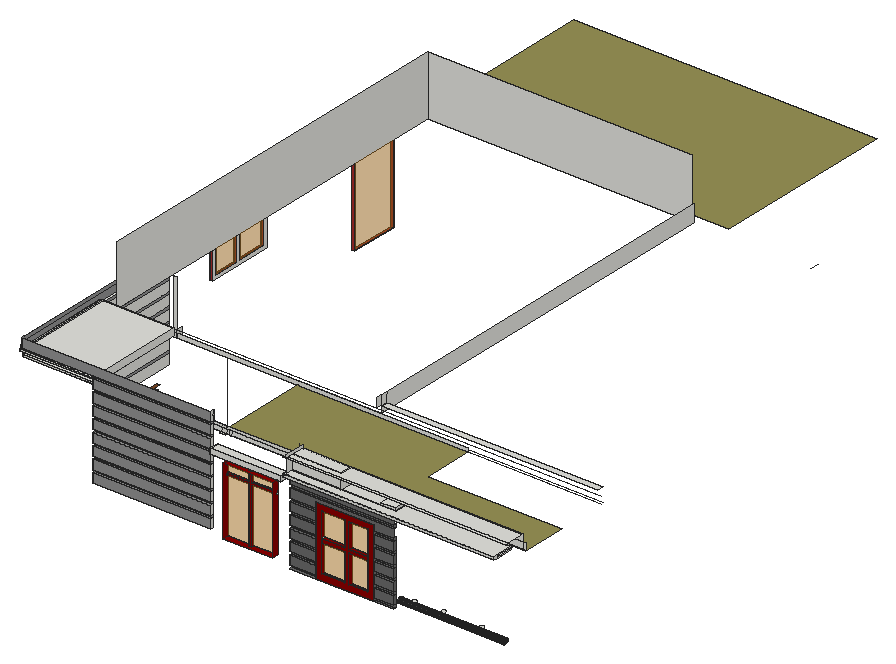
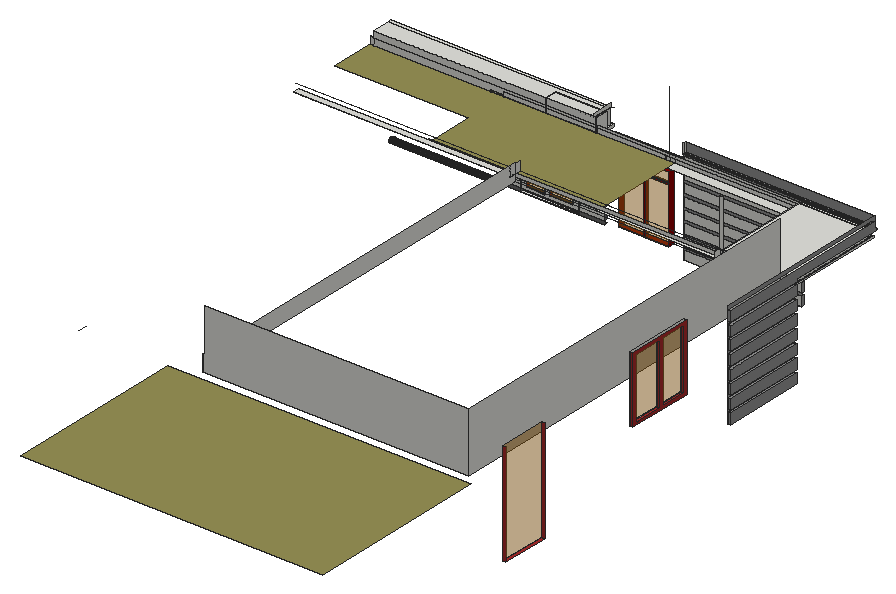
# SketchUp Ruby script. Lengths in inches.
U = 1.inch
M = Sketchup.active_model
def pt(a) = Geom::Point3d.new(a.map { |v| v * U })
def face(e, loops, mat)
  f = e.add_face(loops[0].map { |a| pt(a) })
  loops[1..].each { |l| e.add_face(l.map { |a| pt(a) }).erase! }
  f.material = f.back_material = mat if mat
  f
end
# faces: each face lists its corners as indices into pts; further lists are holes
def faces(e, pts, list, mat = nil) = list.each { |f| face(e, (f[0].is_a?(Array) ? f : [f]).map { |l| l.map { |i| pts[i] } }, mat) }
# xy, xz, yz: faces in a plane at the given z, y or x. An outline is a flat list of corners, or four numbers for a rectangle; further outlines are holes
def ring(l) = l.size == 4 ? [[l[0], l[1]], [l[2], l[1]], [l[2], l[3]], [l[0], l[3]]] : l.each_slice(2).to_a
def flat(e, list, mat, &to3) = list.each { |f| face(e, (f[0].is_a?(Array) ? f : [f]).map { |l| ring(l).map { |u, v| to3.(u, v) } }, mat) }
def xy(e, z, list, mat = nil) = flat(e, list, mat) { |x, y| [x, y, z] }
def xz(e, y, list, mat = nil) = flat(e, list, mat) { |x, z| [x, y, z] }
def yz(e, x, list, mat = nil) = flat(e, list, mat) { |y, z| [x, y, z] }
def lines(e, pts, list) = list.each { |a, b| e.add_line(pt(pts[a]), pt(pts[b])) }
# prism: a flat outline (further loops are holes) pulled along v
def prism(e, loops, v, mat = nil)
  f = face(e, loops, mat); d = Geom::Vector3d.new(v.map { |x| x * U })
  f.pushpull(f.normal.samedirection?(d) ? d.length : -d.length)
end
def box(e, o, s, mat = nil) = prism(e, [[o, [o[0] + s[0], o[1], o[2]], [o[0] + s[0], o[1] + s[1], o[2]], [o[0], o[1] + s[1], o[2]]]], [0, 0, s[2]], mat)
def at(x, y, z, deg = 0) = Geom::Transformation.translation(pt([x, y, z])) * Geom::Transformation.rotation(ORIGIN, Z_AXIS, deg.degrees)
def axes(o, x, y, z) = Geom::Transformation.new([*x, 0, *y, 0, *z, 0, *pt(o).to_a, 1])
def part(name) = M.definitions.add(name)
# library, detail: a bought-in or finely detailed component or shape, given as its bounding box
def library(name, o, s) = part(name).tap { |d| box(d.entities, o, s) }
def detail(e, o, s) = box(e.add_group.entities, o, s)
def put(e, d, t, mat = nil) = e.add_instance(d, t).tap { |i| i.material = mat if mat }
def group(e, t, mat = nil) = e.add_group.tap { |g| g.transformation = t; g.material = mat if mat }.entities
root = M.entities
M.materials.add("[0018_Brown]").color = [165, 42, 42]
M.materials.add("[0021_DarkRed]").color = [139, 0, 0]
M.materials.add("[0038_Orange]").color = [255, 165, 0]
M.materials.add("[0057_DarkKhaki]").color = [150, 145, 85]
M.materials.add("[0134_DimGray]").color = [105, 105, 105]
M.materials.add("[0137_Black]").color = [71, 71, 71]
M.materials.add("[Color M05]").color = [145, 145, 145]
M.materials.add("[Translucent Glass Gray]").color = [191, 123, 24]
M.materials["[Translucent Glass Gray]"].alpha = 0.5
M.materials.add("[Wood Veneer 01]").color = [120, 70, 37]
xy(root,274.6875,[[286.17,7.0625,335.53,10.0625],[335.53,7.0625,390.0625,10.0625]],"[0134_DimGray]")
xy(root,274.97,[[312.43,7.0625,370.43,10.0625]])
xy(root,276.08,[[8.875,431.78,11.875,479.72]],"[0018_Brown]")
xy(root,276.32,[[8.875,116.75,11.875,199.5]],"[Color M05]")
xy(root,276.55,[[82.85,15.1875,200.79,18.1875]])
xy(root,278.27,[[370.43,7.0625,390.0625,10.0625]])
xy(root,278.27,[[286.17,7.0625,312.43,10.0625]],"[0134_DimGray]")
xy(root,278.86,[[242.99,10.1875,245.59,12.1875]])
xy(root,278.86,[[220.5625,6.1875,270.625,6.1875,270.625,12.1875,245.59,12.1875,245.59,10.1875,242.99,10.1875,242.99,12.1875,220.5625,12.1875]],"[0021_DarkRed]")
xy(root,280.97,[[318.43,7.0625,341.43,10.0625],[345.85,7.0625,364.43,10.0625]],"[0021_DarkRed]")
xy(root,285.65,[[82.85,15.1875,200.79,18.1875]],"[Color M05]")
xy(root,286.4,[[8.875,116.75,11.875,199.5]],"[Color M05]")
xy(root,286.45,[[407.42,9.5,407.89,9.5625,408.33,9.74,408.7,10.03,408.99,10.41,409.17,10.84,409.23,11.3125,409.17,11.78,408.99,12.22,408.7,12.6,408.33,12.88,407.89,13.0625,407.42,13.125,406.95,13.0625,406.51,12.88,406.14,12.6,405.85,12.22,405.67,11.78,405.61,11.3125,405.67,10.84,405.85,10.41,406.14,10.03,406.51,9.74,406.95,9.5625]])
xy(root,286.6875,[[286.17,7.0625,312.43,10.0625],[370.43,7.0625,390.0625,10.0625]],"[0134_DimGray]")
xy(root,287.08,[[474.86,9.5,475.33,9.5625,475.76,9.74,476.14,10.03,476.43,10.41,476.61,10.84,476.67,11.3125,476.61,11.78,476.43,12.22,476.14,12.6,475.76,12.88,475.33,13.0625,474.86,13.125,474.39,13.0625,473.95,12.88,473.58,12.6,473.29,12.22,473.11,11.78,473.04,11.3125,473.11,10.84,473.29,10.41,473.58,10.03,473.95,9.74,474.39,9.5625]])
xy(root,287.52,[[437.11,9.5,437.58,9.5625,438.01,9.74,438.39,10.03,438.68,10.41,438.86,10.84,438.92,11.3125,438.86,11.78,438.68,12.22,438.39,12.6,438.01,12.88,437.58,13.0625,437.11,13.125,436.64,13.0625,436.2,12.88,435.83,12.6,435.54,12.22,435.36,11.78,435.29,11.3125,435.36,10.84,435.54,10.41,435.83,10.03,436.2,9.74,436.64,9.5625]])
xy(root,288.55,[[82.85,15.1875,200.79,18.1875]])
xy(root,289.44,[[8.875,116.75,11.875,199.5]],"[Color M05]")
xy(root,290.27,[[370.43,7.0625,390.0625,10.0625]])
xy(root,290.27,[[286.17,7.0625,312.43,10.0625]],"[0134_DimGray]")
xy(root,297.65,[[82.85,15.1875,200.79,18.1875]],"[Color M05]")
xy(root,298.6875,[[286.17,7.0625,312.43,10.0625],[370.43,7.0625,390.0625,10.0625]],"[0134_DimGray]")
xy(root,299.53,[[8.875,116.75,11.875,199.5]],"[Color M05]")
xy(root,300.55,[[82.85,15.1875,200.79,18.1875]])
xy(root,302.27,[[286.17,7.0625,312.43,10.0625],[370.43,7.0625,390.0625,10.0625]],"[0134_DimGray]")
xy(root,302.57,[[8.875,116.75,11.875,199.5]],"[Color M05]")
xy(root,309.43,[[318.43,7.0625,341.43,10.0625],[345.85,7.0625,364.43,10.0625]])
xy(root,309.65,[[82.85,15.1875,200.79,18.1875]],"[Color M05]")
xy(root,310.6875,[[286.17,7.0625,312.43,10.0625],[370.43,7.0625,390.0625,10.0625]],"[0134_DimGray]")
xy(root,312.55,[[82.85,15.1875,200.79,18.1875]])
xy(root,312.65,[[8.875,116.75,11.875,199.5]],"[Color M05]")
xy(root,312.85,[[318.43,7.0625,341.43,10.0625],[345.85,7.0625,364.43,10.0625]],"[0021_DarkRed]")
xy(root,314.27,[[286.17,7.0625,312.43,10.0625],[370.43,7.0625,390.0625,10.0625]],"[0134_DimGray]")
xy(root,315.69,[[8.875,116.75,11.875,199.5]],"[Color M05]")
xy(root,321.65,[[82.85,15.1875,200.79,18.1875]],"[Color M05]")
xy(root,322.6875,[[286.17,7.0625,312.43,10.0625],[370.43,7.0625,390.0625,10.0625]],"[0134_DimGray]")
xy(root,324,[[79.85,66.65,82.85,96.65]])
xy(root,324.55,[[82.85,15.1875,200.79,18.1875]],"[Color M05]")
xy(root,325.78,[[8.875,116.75,11.875,199.5]],"[Color M05]")
xy(root,326.27,[[286.17,7.0625,312.43,10.0625],[370.43,7.0625,390.0625,10.0625]],"[0134_DimGray]")
xy(root,327,[[79.85,63.65,82.85,99.65]],"[Wood Veneer 01]")
xy(root,327.4,[[8.875,254.47,11.875,321.35]],"[0018_Brown]")
xy(root,328.82,[[8.875,116.75,11.875,199.5]],"[Color M05]")
xy(root,330.4,[[8.875,257.47,11.875,284.61],[8.875,287.91,11.875,318.35]],"[0018_Brown]")
xy(root,333.65,[[82.85,15.1875,200.79,18.1875]],"[Color M05]")
xy(root,334.3,[[220.5625,10.1875,242.99,12.1875],[245.59,10.1875,270.625,12.1875]],"[0021_DarkRed]")
xy(root,334.6875,[[286.17,7.0625,312.43,10.0625],[370.43,7.0625,390.0625,10.0625]],"[0134_DimGray]")
xy(root,336.28,[[220.5625,10.1875,242.99,12.1875],[245.59,10.1875,270.625,12.1875]],"[0021_DarkRed]")
xy(root,336.55,[[82.85,15.1875,200.79,18.1875]],"[Color M05]")
xy(root,337.9,[[318.43,7.0625,341.43,10.0625],[345.85,7.0625,364.43,10.0625]])
xy(root,338.27,[[286.17,7.0625,312.43,10.0625],[370.43,7.0625,390.0625,10.0625]],"[0134_DimGray]")
xy(root,338.9,[[8.875,116.75,11.875,199.5]],"[Color M05]")
xy(root,341.94,[[8.875,116.75,11.875,199.5]],"[Color M05]")
xy(root,343.9,[[312.43,7.0625,370.43,10.0625]])
xy(root,345.65,[[82.85,15.1875,200.79,18.1875]],"[Color M05]")
xy(root,346.36,[[242.99,10.1875,245.59,12.1875]])
xy(root,346.36,[[220.5625,6.1875,220.5625,12.1875,242.99,12.1875,242.99,10.1875,245.59,10.1875,245.59,12.1875,270.625,12.1875,270.625,6.1875]],"[0021_DarkRed]")
xy(root,346.6875,[[286.17,7.0625,390.0625,10.0625]],"[0134_DimGray]")
xy(root,348.55,[[82.85,15.1875,200.79,18.1875]],"[Color M05]")
xy(root,350.27,[[286.17,7.0625,390.0625,10.0625]],"[0134_DimGray]")
xy(root,352.03,[[8.875,116.75,11.875,199.5]],"[Color M05]")
xy(root,352.16,[[209.95,3.1875,214.5625,12.1875],[276.625,3.1875,278.01,12.1875],[278.01,3.1875,280.45,12.1875],[280.45,3.1875,280.75,12.1875]])
xy(root,352.36,[[214.5625,3.1875,276.625,6.1875],[214.5625,6.1875,276.625,12.1875]])
xy(root,355.07,[[8.875,116.75,11.875,199.5]])
xy(root,357.35,[[209.95,3.1875,280.45,12.1875]])
xy(root,357.65,[[82.85,15.1875,200.79,18.1875]],"[Color M05]")
xy(root,358.6875,[[284.41,1.0625,284.41,10.0625,286.17,10.0625,286.17,7.0625,390.0625,7.0625,390.0625,22.0625,495.71,22.0625,495.71,1.0625],[286.17,7.0625,286.99,10.0625],[286.99,7.0625,335.53,10.0625],[335.53,7.0625,375.29,10.0625],[375.29,7.0625,390.0625,10.0625],
  [284.41,10.0625,335.53,22.0625],[335.53,10.0625,390.0625,22.0625]])
xy(root,360.55,[[82.85,15.1875,200.79,18.1875]],"[Color M05]")
xy(root,361.64,[[285.64,4.0625,497.49,22.0625]])
xy(root,361.6875,[[284.41,1.0625,495.71,1.0625,495.71,22.0625,390.0625,22.0625,390.0625,10.0625,284.41,10.0625]])
xy(root,363,[[206.66,19.6875,211.87,22.0625],[211.87,21.8125,216.79,22.0625],[86.03,22.0625,206.66,31.8125],[86.03,116.75,206.66,119.6875]])
xy(root,363,[[206.66,22.0625,206.66,116.75,376.99,116.75,376.99,66.25,510.6875,66.25,510.6875,22.0625],[11.875,520.875,314.375,705.1875]],"[0057_DarkKhaki]")
xy(root,363.17,[[11.875,22.0625,20.6875,32.5]])
xy(root,363.37,[[10.5625,18.1875,82.85,116.75]])
xy(root,363.92,[[375.29,10.0625,390.0625,22.0625]])
xy(root,364.96,[[10.5625,18.1875,82.85,18.1875,82.85,21.1875,11.875,21.1875,11.875,116.75,10.5625,116.75]])
xy(root,365.15,[[8.875,116.75,11.875,199.5]],"[Color M05]")
xy(root,368.19,[[8.875,116.75,11.875,199.5]])
xy(root,369.18,[[10.1875,15.5625,10.1875,116.75,11.875,116.75,11.875,21.1875,82.85,21.1875,82.85,15.5625]])
xy(root,369.65,[[82.85,15.1875,200.79,18.1875]],"[Color M05]")
xy(root,369.99,[[285.29,122.75,286.17,128.75],[286.17,122.75,501.6875,128.75]])
xy(root,370.55,[[10.1875,15.5625,82.85,18.1875],[8.875,18.1875,10.1875,116.75],[10.1875,18.1875,11.875,21.1875],[11.875,18.1875,82.85,21.1875],[10.1875,21.1875,11.875,21.75],
  [11.875,21.1875,82.85,21.75],[10.1875,21.75,11.875,116.75],[11.875,21.75,82.85,116.75]])
xy(root,372.55,[[8.875,18.1875,11.875,19],[11.875,18.1875,200.79,19]])
xy(root,372.55,[[11.875,15.1875,200.79,18.1875]],"[Color M05]")
xy(root,376.42,[[286.99,1.0625,507.04,4.0625],[285.64,4.0625,286.99,10.0625],[286.99,4.0625,507.04,4.0625,507.04,22.0625,335.53,22.0625,335.53,10.0625,286.99,10.0625],[284.41,10.0625,285.64,22.0625],[285.64,10.0625,286.99,22.0625],
  [286.99,10.0625,335.53,22.0625]])
xz(root,1.0625,[[284.41,358.6875,495.71,361.64],[284.41,361.64,285.29,361.6875],[285.29,361.64,286.17,361.6875],[286.17,361.64,286.99,361.6875],[286.99,361.64,495.71,361.6875]])
xz(root,3.1875,[[209.95,352.16,214.5625,352.16,214.5625,352.36,276.625,352.36,276.625,352.16,280.45,352.16,280.45,357.35,209.95,357.35]])
xz(root,7.0625,[[[312.43,274.97,370.43,343.9],[318.43,280.97,318.43,337.9,341.43,337.9,341.43,312.85,318.43,312.85,318.43,309.43,341.43,309.43,341.43,280.97],[345.85,280.97,345.85,309.43,364.43,309.43,364.43,312.85,345.85,312.85,345.85,337.9,364.43,337.9,364.43,280.97]]],"[0021_DarkRed]")
xz(root,7.0625,[[286.17,278.27,312.43,286.6875],[370.43,278.27,390.0625,286.6875],[286.17,290.27,312.43,298.6875],[370.43,290.27,390.0625,298.6875],[286.17,302.27,312.43,310.6875],
  [370.43,302.27,390.0625,310.6875],[286.17,314.27,312.43,322.6875],[370.43,314.27,390.0625,322.6875],[286.17,326.27,312.43,334.6875],[370.43,326.27,390.0625,334.6875],
  [286.17,338.27,312.43,338.27,312.43,343.9,370.43,343.9,370.43,338.27,390.0625,338.27,390.0625,346.6875,286.17,346.6875],[286.17,350.27,390.0625,358.6875]],"[0134_DimGray]")
xz(root,10.0625,[[286.17,278.27,312.43,286.6875],[312.43,278.27,370.43,278.27,370.43,286.6875,364.43,286.6875,364.43,280.97,345.85,280.97,345.85,286.6875,341.43,286.6875,341.43,280.97,318.43,280.97,318.43,286.6875,312.43,286.6875],[370.43,278.27,390.0625,286.6875],[286.17,290.27,312.43,298.6875],[312.43,290.27,318.43,298.6875],
  [341.43,290.27,345.85,298.6875],[364.43,290.27,370.43,298.6875],[370.43,290.27,390.0625,298.6875],[286.17,302.27,312.43,310.6875],[312.43,302.27,318.43,310.6875],
  [341.43,302.27,345.85,302.27,345.85,309.43,364.43,309.43,364.43,310.6875,318.43,310.6875,318.43,309.43,341.43,309.43],[364.43,302.27,370.43,310.6875],[370.43,302.27,390.0625,310.6875],[286.17,314.27,312.43,322.6875],[312.43,314.27,318.43,322.6875],
  [341.43,314.27,345.85,322.6875],[364.43,314.27,370.43,322.6875],[370.43,314.27,390.0625,322.6875],[286.17,326.27,312.43,334.6875],[312.43,326.27,318.43,334.6875],
  [341.43,326.27,345.85,334.6875],[364.43,326.27,370.43,334.6875],[370.43,326.27,390.0625,334.6875],[312.43,338.27,370.43,343.9],[284.41,358.6875,286.17,361.6875],
  [286.17,358.6875,286.99,361.6875],[286.99,358.6875,335.53,361.6875],[335.53,358.6875,375.29,361.6875],[375.29,358.6875,390.0625,361.6875],[284.41,361.6875,335.53,376.42],
  [375.29,361.6875,390.0625,363.92]])
xz(root,10.0625,[[286.17,274.6875,390.0625,274.6875,390.0625,278.27,370.43,278.27,370.43,274.97,312.43,274.97,312.43,278.27,286.17,278.27],[286.17,286.6875,312.43,290.27],[370.43,286.6875,390.0625,290.27],[286.17,298.6875,312.43,302.27],[370.43,298.6875,390.0625,302.27],
  [286.17,310.6875,312.43,314.27],[370.43,310.6875,390.0625,314.27],[286.17,322.6875,312.43,326.27],[370.43,322.6875,390.0625,326.27],[286.17,334.6875,312.43,338.27],
  [370.43,334.6875,390.0625,338.27],[286.17,346.6875,390.0625,350.27]],"[0134_DimGray]")
xz(root,10.0625,[[318.43,280.97,341.43,309.43],[345.85,280.97,364.43,309.43],[318.43,312.85,341.43,337.9],[345.85,312.85,364.43,337.9]],"[Translucent Glass Gray]")
xz(root,10.1875,[[242.99,278.86,245.59,278.86,245.59,334.3,270.625,334.3,270.625,336.28,245.59,336.28,245.59,346.36,242.99,346.36,242.99,336.28,220.5625,336.28,220.5625,334.3,242.99,334.3]],"[0021_DarkRed]")
xz(root,12.1875,[[214.5625,352.16,276.625,352.36]])
xz(root,12.1875,[[220.5625,278.86,242.99,334.3],[245.59,278.86,270.625,334.3],[220.5625,336.28,242.99,346.36],[245.59,336.28,270.625,346.36]],"[Translucent Glass Gray]")
xz(root,15.1875,[[82.85,276.55,200.79,285.65],[82.85,288.55,200.79,297.65],[82.85,300.55,200.79,309.65],[82.85,312.55,200.79,321.65],[82.85,324.55,200.79,333.65],
  [82.85,336.55,200.79,345.65],[82.85,348.55,200.79,357.65],[82.85,360.55,200.79,369.65],[11.875,372.55,200.79,381.65]],"[Color M05]")
xz(root,15.5625,[[10.1875,369.18,82.85,370.55]])
xz(root,18.1875,[[82.85,276.55,200.79,285.65],[82.85,288.55,200.79,297.65],[82.85,300.55,200.79,309.65],[82.85,312.55,200.79,321.65],[82.85,324.55,200.79,333.65],
  [82.85,336.55,200.79,345.65],[82.85,348.55,200.79,357.65],[82.85,360.55,200.79,369.65],[10.5625,363.37,11.875,364.96],[11.875,363.37,82.85,364.96]])
xz(root,18.1875,[[82.85,285.65,200.79,288.55],[82.85,297.65,200.79,300.55],[82.85,309.65,200.79,312.55],[82.85,321.65,200.79,324.55],[82.85,333.65,200.79,336.55],
  [82.85,345.65,200.79,348.55],[82.85,357.65,200.79,360.55],[82.85,369.65,200.79,369.65,200.79,372.55,8.875,372.55,8.875,370.55,82.85,370.55]],"[Color M05]")
xz(root,19,[[8.875,372.55,11.875,378.28]],"[Color M05]")
xz(root,21.1875,[[11.875,364.96,82.85,369.18],[11.875,369.18,82.85,370.55]])
xz(root,22.0625,[[284.41,358.6875,284.41,363,285.64,363,285.64,361.64,335.53,361.64,335.53,358.6875],[335.53,358.6875,375.29,361.64],[375.29,358.6875,376.99,361.64],[376.99,358.6875,390.0625,361.64],[390.0625,358.6875,494.09,361.64],
  [494.09,358.6875,495.71,361.64],[285.64,361.64,335.53,363],[335.53,361.64,375.29,363],[375.29,361.64,376.99,363],[376.99,361.64,390.0625,363],
  [390.0625,361.64,494.09,361.6875],[494.09,361.64,495.71,361.6875],[390.0625,361.6875,494.09,363],[86.03,363,206.66,367],[206.66,363,211.87,363,211.79,367,206.66,367],
  [211.87,363,211.79,367,214.3,367,214.3,363],[214.3,363,216.79,367],[216.79,363,284.41,367],[284.41,363,285.64,367],[285.64,363,335.53,367],
  [335.53,363,335.53,367,376.99,367,376.99,363.92,375.29,363.92,375.29,363],[390.0625,363,390.0625,363.92,376.99,363.92,376.99,367,335.53,367,335.53,369.99,507.04,369.99,507.04,363],[375.29,363,376.99,363.92],[375.29,363,390.0625,363.92],[376.99,363,390.0625,363.92],
  [507.04,363,510.6875,369.99],[86.03,367,206.66,369.99],[206.66,367,206.66,369.99,211.73,369.99,211.79,367],[211.79,367,211.73,369.99,284.41,369.99,284.41,367],[284.41,367,285.64,369.99],
  [285.64,367,335.53,369.99],[284.41,369.99,285.64,376.42],[285.64,369.99,335.53,376.42],[335.53,369.99,507.04,376.42]])
xz(root,116.75,[[82.85,363,86.03,367],[86.03,363,376.99,367],[8.875,363.37,10.5625,364.96],[10.5625,363.37,11.875,364.96],[11.875,363.37,82.85,370.55],
  [8.875,364.96,11.875,365.15],[82.85,367,86.03,369.99],[8.875,368.19,11.875,369.18],[8.875,369.18,10.1875,370.55],[10.1875,369.18,11.875,370.55],
  [82.85,369.99,86.03,417.65]])
xz(root,116.75,[[8.875,276.32,11.875,286.4],[8.875,289.44,11.875,299.53],[8.875,302.57,11.875,312.65],[8.875,315.69,11.875,325.78],[8.875,328.82,11.875,338.9],
  [8.875,341.94,11.875,352.03],[8.875,355.07,11.875,363.37]],"[Color M05]")
xz(root,122.75,[[285.29,369.99,286.17,379.43]])
xz(root,199.5,[[8.875,276.32,11.875,286.4],[8.875,289.44,11.875,299.53],[8.875,302.57,11.875,312.65],[8.875,315.69,11.875,325.78],[8.875,328.82,11.875,338.9],
  [8.875,341.94,11.875,352.03],[8.875,355.07,11.875,365.15],[8.875,368.19,11.875,378.28]],"[Color M05]")
xz(root,254.47,[[8.875,327.4,11.875,394.28]],"[0018_Brown]")
xz(root,257.47,[[8.875,330.4,11.875,391.28]],"[0018_Brown]")
xz(root,284.61,[[8.875,330.4,11.875,391.28]],"[0018_Brown]")
xz(root,287.91,[[8.875,330.4,11.875,391.28]],"[0018_Brown]")
xz(root,318.35,[[8.875,330.4,11.875,391.28]],"[0018_Brown]")
xz(root,321.35,[[8.875,327.4,11.875,394.28]],"[0018_Brown]")
xz(root,431.78,[[8.875,276.08,11.875,379.4]],"[0018_Brown]")
xz(root,479.72,[[8.875,276.08,11.875,379.4]],"[0018_Brown]")
xz(root,511.875,[[20.875,363,20.875,423,284.05,423,284.05,379.43,286.17,379.43,286.17,363]])
yz(root,8.875,[[[254.47,327.4,321.35,394.28],[287.91,330.4,318.35,391.28],[257.47,330.4,284.61,391.28]]],"[0018_Brown]")
yz(root,8.875,[[116.75,276.32,199.5,286.4],[116.75,289.44,199.5,299.53],[116.75,302.57,199.5,312.65],[116.75,315.69,199.5,325.78],[116.75,328.82,199.5,338.9],
  [116.75,341.94,199.5,352.03],[116.75,355.07,199.5,365.15],[116.75,368.19,116.75,370.55,18.1875,370.55,18.1875,372.55,19,372.55,19,378.28,199.5,378.28,199.5,368.19]],"[Color M05]")
yz(root,10.1875,[[15.5625,369.18,116.75,370.55]])
yz(root,10.5625,[[18.1875,363.37,116.75,364.96]])
yz(root,11.875,[[116.75,276.32,199.5,286.4],[116.75,289.44,199.5,299.53],[116.75,302.57,199.5,312.65],[116.75,315.69,199.5,325.78],[[254.47,327.4,321.35,394.28],[287.91,330.4,318.35,391.28],[257.47,330.4,284.61,391.28]],
  [116.75,328.82,199.5,338.9],[116.75,341.94,199.5,352.03],[116.75,355.07,199.5,365.15],[21.1875,364.96,116.75,365.15],[21.1875,365.15,116.75,369.18],
  [21.1875,369.18,116.75,370.55]])
yz(root,11.875,[[116.75,286.4,199.5,289.44],[116.75,299.53,199.5,302.57],[116.75,312.65,199.5,315.69],[116.75,325.78,199.5,328.82],[116.75,338.9,199.5,341.94],
  [116.75,352.03,199.5,355.07],[116.75,365.15,199.5,368.19],[15.1875,372.55,15.1875,381.65,18.1875,381.65,18.1875,381.32,199.5,381.32,199.5,378.28,19,378.28,19,372.55]],"[Color M05]")
yz(root,11.875,[[431.78,276.08,479.72,379.4],[257.47,330.4,284.61,391.28],[287.91,330.4,318.35,391.28]],"[Translucent Glass Gray]")
yz(root,20.875,[[122.75,363,511.875,423]])
yz(root,82.85,[[18.1875,363.37,21.1875,364.96],[21.1875,363.37,116.75,370.55],[15.1875,369.18,15.5625,369.65],[15.5625,369.18,18.1875,369.65],[18.1875,369.18,21.1875,370.55],
  [15.5625,369.65,18.1875,370.55]])
yz(root,82.85,[[66.65,282.49,96.65,284.19],[66.65,293.24,96.65,294.94],[66.65,303.99,96.65,305.69],[66.65,314.74,96.65,316.44]],"[0038_Orange]")
yz(root,82.85,[[15.1875,276.55,18.1875,285.65],[15.1875,288.55,18.1875,297.65],[15.1875,300.55,18.1875,309.65],[15.1875,312.55,18.1875,321.65],[15.1875,324.55,18.1875,333.65],
  [15.1875,336.55,18.1875,345.65],[15.1875,348.55,18.1875,357.65],[15.1875,360.55,18.1875,363.37],[15.1875,363.37,18.1875,364.96],[15.1875,364.96,18.1875,369.18],
  [18.1875,364.96,21.1875,369.18]],"[Color M05]")
yz(root,82.85,[[66.65,284.19,96.65,293.24],[66.65,294.94,96.65,303.99],[66.65,305.69,96.65,314.74],[66.65,316.44,96.65,324]],"[Wood Veneer 01]")
yz(root,86.03,[[116.75,363,122.9375,369.99]])
yz(root,200.79,[[15.1875,276.55,18.1875,285.65],[15.1875,288.55,18.1875,297.65],[15.1875,300.55,18.1875,309.65],[15.1875,312.55,18.1875,321.65],[15.1875,324.55,18.1875,333.65],
  [15.1875,336.55,18.1875,345.65],[15.1875,348.55,18.1875,357.65],[15.1875,360.55,18.1875,369.65],[15.1875,372.55,18.1875,381.65],[18.1875,372.55,19,381.65]])
yz(root,209.95,[[3.1875,352.16,12.1875,357.35]])
yz(root,214.5625,[[3.1875,352.16,6.1875,352.36],[6.1875,352.16,12.1875,352.36]])
yz(root,220.5625,[[10.1875,334.3,12.1875,336.28]])
yz(root,220.5625,[[6.1875,278.86,12.1875,278.86,12.1875,334.3,10.1875,334.3,10.1875,336.28,12.1875,336.28,12.1875,346.36,6.1875,346.36]],"[0021_DarkRed]")
yz(root,242.99,[[10.1875,278.86,12.1875,334.3],[10.1875,336.28,12.1875,346.36]],"[0021_DarkRed]")
yz(root,245.59,[[10.1875,278.86,12.1875,334.3],[10.1875,336.28,12.1875,346.36]],"[0021_DarkRed]")
yz(root,270.625,[[10.1875,334.3,12.1875,336.28]])
yz(root,270.625,[[6.1875,278.86,6.1875,346.36,12.1875,346.36,12.1875,336.28,10.1875,336.28,10.1875,334.3,12.1875,334.3,12.1875,278.86]],"[0021_DarkRed]")
yz(root,276.625,[[3.1875,352.16,6.1875,352.36],[6.1875,352.16,12.1875,352.36]])
yz(root,280.45,[[3.1875,352.16,12.1875,357.35]])
yz(root,284.41,[[1.0625,358.6875,10.0625,361.6875],[10.0625,358.6875,22.0625,376.42]])
yz(root,285.29,[[116.75,369.99,122.75,379.43]])
yz(root,285.64,[[4.0625,361.64,22.0625,376.42]])
yz(root,286.17,[[7.0625,350.27,10.0625,358.6875],[122.75,363,511.875,363,511.875,379.43,128.75,379.43,128.75,369.99,122.75,369.99],[122.75,369.99,128.75,379.43]])
yz(root,286.17,[[7.0625,278.27,10.0625,286.6875],[7.0625,290.27,10.0625,298.6875],[7.0625,302.27,10.0625,310.6875],[7.0625,314.27,10.0625,322.6875],[7.0625,326.27,10.0625,334.6875],
  [7.0625,338.27,10.0625,346.6875]],"[0134_DimGray]")
yz(root,286.99,[[1.0625,376.42,22.0625,379.43]])
yz(root,312.43,[[7.0625,278.27,10.0625,286.6875],[7.0625,290.27,10.0625,298.6875],[7.0625,302.27,10.0625,310.6875],[7.0625,314.27,10.0625,322.6875],[7.0625,326.27,10.0625,334.6875],
  [7.0625,338.27,10.0625,343.9]])
yz(root,312.43,[[7.0625,274.97,10.0625,278.27],[7.0625,286.6875,10.0625,290.27],[7.0625,298.6875,10.0625,302.27],[7.0625,310.6875,10.0625,314.27],[7.0625,322.6875,10.0625,326.27],
  [7.0625,334.6875,10.0625,338.27]],"[0134_DimGray]")
yz(root,318.43,[[7.0625,309.43,10.0625,312.85]])
yz(root,318.43,[[7.0625,280.97,10.0625,309.43],[7.0625,312.85,10.0625,337.9]],"[0021_DarkRed]")
yz(root,335.53,[[10.0625,358.6875,22.0625,376.42]])
yz(root,341.43,[[7.0625,280.97,10.0625,309.43],[7.0625,312.85,10.0625,337.9]],"[0021_DarkRed]")
yz(root,345.85,[[7.0625,280.97,10.0625,309.43],[7.0625,312.85,10.0625,337.9]],"[0021_DarkRed]")
yz(root,364.43,[[7.0625,309.43,10.0625,312.85]])
yz(root,364.43,[[7.0625,280.97,10.0625,309.43],[7.0625,312.85,10.0625,337.9]],"[0021_DarkRed]")
yz(root,370.43,[[7.0625,278.27,10.0625,286.6875],[7.0625,290.27,10.0625,298.6875],[7.0625,302.27,10.0625,310.6875],[7.0625,314.27,10.0625,322.6875],[7.0625,326.27,10.0625,334.6875],
  [7.0625,338.27,10.0625,343.9]])
yz(root,370.43,[[7.0625,274.97,10.0625,278.27],[7.0625,286.6875,10.0625,290.27],[7.0625,298.6875,10.0625,302.27],[7.0625,310.6875,10.0625,314.27],[7.0625,322.6875,10.0625,326.27],
  [7.0625,334.6875,10.0625,338.27]],"[0134_DimGray]")
yz(root,390.0625,[[10.0625,358.6875,22.0625,361.6875],[10.0625,361.6875,22.0625,363.92]])
yz(root,390.0625,[[7.0625,278.27,10.0625,286.6875],[7.0625,290.27,10.0625,298.6875],[7.0625,302.27,10.0625,310.6875],[7.0625,314.27,10.0625,322.6875],[7.0625,326.27,10.0625,334.6875]],"[0134_DimGray]")
yz(root,495.71,[[1.0625,358.6875,4.0625,361.6875],[4.0625,358.6875,10.0625,361.6875],[10.0625,358.6875,22.0625,361.6875]])
p = [[390.0625,14.55,277.06],[390.0625,15.21,276.97],[495.71,15.21,276.97],[495.71,14.55,277.06],[390.0625,15.87,277.06],[495.71,15.87,277.06],
  [390.0625,13.93,277.3125],[495.71,13.93,277.3125],[390.0625,16.49,277.3125],[495.71,16.49,277.3125],[390.0625,13.4,277.72],[495.71,13.4,277.72],
  [390.0625,17.02,277.72],[495.71,17.02,277.72],[390.0625,12.99,278.25],[495.71,12.99,278.25],[390.0625,17.43,278.25],[495.71,17.43,278.25],
  [390.0625,12.73,278.87],[495.71,12.73,278.87],[390.0625,17.68,278.87],[495.71,17.68,278.87],[390.0625,12.65,279.53],[495.71,12.65,279.53],
  [390.0625,17.77,279.53],[495.71,17.77,279.53],[390.0625,12.73,280.2],[495.71,12.73,280.2],[390.0625,17.68,280.2],[495.71,17.68,280.2],
  [390.0625,12.99,280.8125],[495.71,12.99,280.8125],[390.0625,17.43,280.8125],[495.71,17.43,280.8125],[390.0625,13.4,281.34],[495.71,13.4,281.34],
  [390.0625,17.02,281.34],[495.71,17.02,281.34],[390.0625,13.93,281.75],[495.71,13.93,281.75],[390.0625,16.49,281.75],[495.71,16.49,281.75],
  [390.0625,14.55,282.01],[495.71,14.55,282.01],[390.0625,15.87,282.01],[495.71,15.87,282.01],[390.0625,15.21,282.09],[495.71,15.21,282.09],
  [403.375,511.875,363],[403.375,520.875,363],[285.29,116.75,369.99],[86.03,116.75,369.99],[211.73,22.0625,429.99],[211.73,22.0625,369.99],
  [509.75,116.75,369.99],[206.66,119.6875,363],[509.75,119.6875,363],[86.03,122.75,363],[286.17,122.75,363],[376.99,116.75,363],
  [509.75,116.75,363],[284.41,1.0625,376.42],[284.05,1.0625,376.42],[11.875,21.1875,363.37],[11.875,21.1875,364.96],[284.41,22.0625,376.42],
  [284.41,22.0625,379.43],[285.64,1.0625,376.42],[285.64,4.0625,376.42],[11.875,21.1875,365.15],[11.875,18.1875,365.15],[11.875,18.1875,369.65],
  [82.85,18.1875,369.65],[11.875,18.1875,370.55],[11.875,18.1875,364.96]]
faces(root,p,[[0,1,2,3],[1,4,5,2],[6,0,3,7],[4,8,9,5],[10,6,7,11],[8,12,13,9],[14,10,11,15],[12,16,17,13],
  [18,14,15,19],[16,20,21,17],[22,18,19,23],[20,24,25,21],[26,22,23,27],[24,28,29,25],[30,26,27,31],[28,32,33,29],
  [34,30,31,35],[32,36,37,33],[38,34,35,39],[36,40,41,37],[42,38,39,43],[40,44,45,41],[46,42,43,47],[44,46,47,45]],"[0137_Black]")
lines(root,p,[[48,49],[50,51],[52,53],[54,50],[55,56],[57,58],[59,60],[61,62],[63,64],[65,66],[67,68],[69,70],
  [71,72],[71,73],[74,70]])
